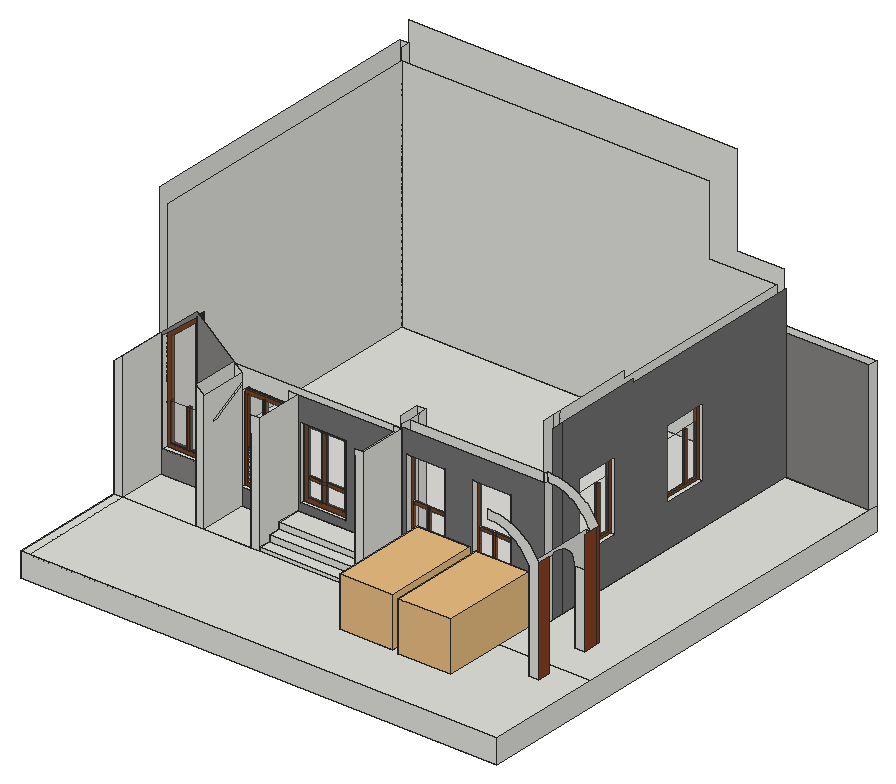
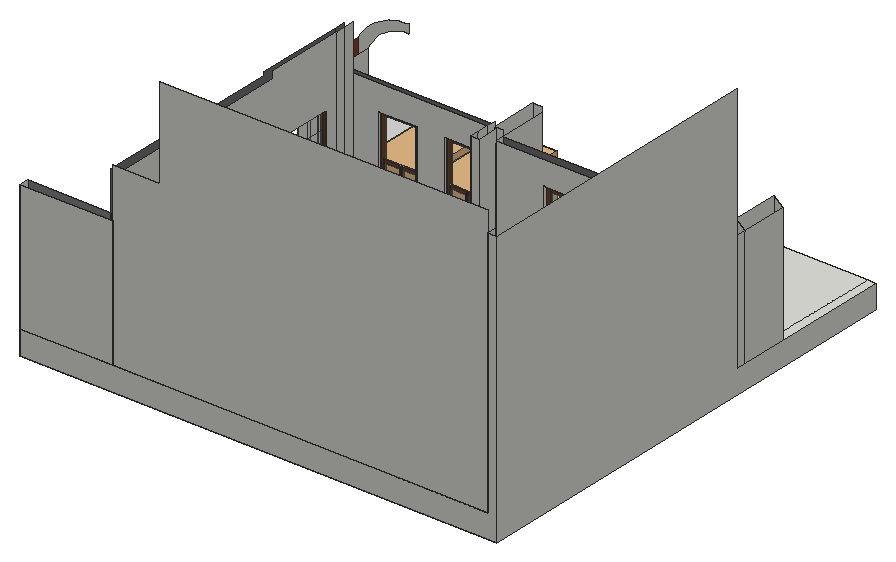
# SketchUp Ruby script. Lengths in inches.
U = 1.inch
M = Sketchup.active_model
def pt(a) = Geom::Point3d.new(a.map { |v| v * U })
def face(e, loops, mat)
  f = e.add_face(loops[0].map { |a| pt(a) })
  loops[1..].each { |l| e.add_face(l.map { |a| pt(a) }).erase! }
  f.material = f.back_material = mat if mat
  f
end
# faces: each face lists its corners as indices into pts; further lists are holes
def faces(e, pts, list, mat = nil) = list.each { |f| face(e, (f[0].is_a?(Array) ? f : [f]).map { |l| l.map { |i| pts[i] } }, mat) }
# xy, xz, yz: faces in a plane at the given z, y or x. An outline is a flat list of corners, or four numbers for a rectangle; further outlines are holes
def ring(l) = l.size == 4 ? [[l[0], l[1]], [l[2], l[1]], [l[2], l[3]], [l[0], l[3]]] : l.each_slice(2).to_a
def flat(e, list, mat, &to3) = list.each { |f| face(e, (f[0].is_a?(Array) ? f : [f]).map { |l| ring(l).map { |u, v| to3.(u, v) } }, mat) }
def xy(e, z, list, mat = nil) = flat(e, list, mat) { |x, y| [x, y, z] }
def xz(e, y, list, mat = nil) = flat(e, list, mat) { |x, z| [x, y, z] }
def yz(e, x, list, mat = nil) = flat(e, list, mat) { |y, z| [x, y, z] }
def lines(e, pts, list) = list.each { |a, b| e.add_line(pt(pts[a]), pt(pts[b])) }
# prism: a flat outline (further loops are holes) pulled along v
def prism(e, loops, v, mat = nil)
  f = face(e, loops, mat); d = Geom::Vector3d.new(v.map { |x| x * U })
  f.pushpull(f.normal.samedirection?(d) ? d.length : -d.length)
end
def box(e, o, s, mat = nil) = prism(e, [[o, [o[0] + s[0], o[1], o[2]], [o[0] + s[0], o[1] + s[1], o[2]], [o[0], o[1] + s[1], o[2]]]], [0, 0, s[2]], mat)
def at(x, y, z, deg = 0) = Geom::Transformation.translation(pt([x, y, z])) * Geom::Transformation.rotation(ORIGIN, Z_AXIS, deg.degrees)
def axes(o, x, y, z) = Geom::Transformation.new([*x, 0, *y, 0, *z, 0, *pt(o).to_a, 1])
def part(name) = M.definitions.add(name)
# library, detail: a bought-in or finely detailed component or shape, given as its bounding box
def library(name, o, s) = part(name).tap { |d| box(d.entities, o, s) }
def detail(e, o, s) = box(e.add_group.entities, o, s)
def put(e, d, t, mat = nil) = e.add_instance(d, t).tap { |i| i.material = mat if mat }
def group(e, t, mat = nil) = e.add_group.tap { |g| g.transformation = t; g.material = mat if mat }.entities
root = M.entities
M.materials.add("Glass Thin Clear 001").color = [243, 240, 240]
M.materials["Glass Thin Clear 001"].alpha = 0.1
M.materials.add("[Brick Tumbled]").color = [135, 132, 132]
M.materials.add("[Color M05]").color = [114, 114, 114]
M.materials.add("[Roofing Tile Spanish]").color = [138, 64, 36]
M.materials.add("[Wood Veneer 01]").color = [120, 70, 37]
c1 = library("2016+Honda+Civic+LX+Sedan",[0.01,0.03,0.02],[16.17,34.46,10.62])
xy(root,-24,[[9.96,0,489.96,478.0625]])
xy(root,0,[[9.96,0,18.96,118.0625],[[18.96,0,489.96,118.0625],[446.88,93.6875,457.27,105.875]],[446.88,93.6875,457.27,105.875],[9.96,118.0625,18.96,166.0625],[18.96,118.0625,91.87,166.0625],
  [91.87,118.0625,156.96,166.0625],[91.87,118.0625,99.96,166.0625],[99.96,118.0625,147.96,166.0625],[147.96,118.0625,156.96,166.0625],[156.96,118.0625,252.96,166.0625],
  [252.96,118.0625,261.96,166.0625],[[261.96,118.0625,489.96,118.0625,489.96,469.0625,405.96,469.0625,405.96,166.0625,261.96,166.0625],[446.88,151.74,457.27,169.5]],[446.88,151.74,457.27,166.0625],[9.96,166.0625,18.96,175.0625],[18.96,166.0625,252.96,175.0625],
  [252.96,166.0625,261.96,196.0625],[252.96,166.0625,405.96,166.0625,405.96,469.0625,396.96,469.0625,396.96,196.0625,252.96,196.0625],[261.96,166.0625,405.96,175.0625],[446.88,166.0625,457.27,169.5],[446.88,166.0625,457.27,169.5],
  [18.96,175.0625,252.96,175.0625,252.96,196.0625,396.96,196.0625,396.96,469.0625,18.96,469.0625],[261.96,175.0625,396.96,187.0625],[396.96,175.0625,405.96,187.0625],[261.96,187.0625,396.96,196.0625],[396.96,187.0625,405.96,469.0625],
  [18.96,469.0625,396.96,478.0625],[396.96,469.0625,489.96,478.0625]])
xy(root,3.4375,[[156.96,118.0625,252.96,129.9375]])
xy(root,9.4375,[[156.96,129.9375,252.96,142.0625]])
xy(root,15.4375,[[156.96,142.0625,252.96,166.0625]])
xy(root,16.69,[[99.96,166.0625,147.96,170.5625],[99.96,173.4375,147.96,175.0625]])
xy(root,16.69,[[99.96,170.5625,147.96,172.375],[99.96,172.375,147.96,173.4375]],"[Wood Veneer 01]")
xy(root,19.54,[[102.81,170.5625,117.68,171.125],[117.68,170.5625,120.35,173.4375],[120.35,170.5625,145.12,171.125]])
xy(root,19.54,[[102.81,171.125,117.68,173.4375],[120.35,171.125,145.12,173.4375]],"[Wood Veneer 01]")
xy(root,22.88,[[159.41,166.0625,204.66,170.5625],[159.41,170.5625,204.66,171.8125],[159.41,171.8125,204.66,172.375],[159.41,172.375,204.66,175.0625]])
xy(root,23.7,[[21.04,166.0625,54.79,170.5625],[21.04,173.875,54.79,175.0625]])
xy(root,23.7,[[21.04,170.5625,54.79,171.0625],[21.04,171.0625,54.79,173.0625],[21.04,173.0625,54.79,173.875]],"[Wood Veneer 01]")
xy(root,27.23,[[177.76,170.5625,182.03,172.375]])
xy(root,27.23,[[163.76,170.5625,177.76,170.875],[182.03,170.5625,200.3125,170.875],[163.76,170.875,177.76,172.375],[182.03,170.875,200.3125,172.375]],"[Wood Veneer 01]")
xy(root,27.76,[[41.61,170.5625,44.06,171.0625],[41.61,171.0625,44.06,173.875]])
xy(root,27.76,[[25.1,170.5625,41.61,171.0625],[44.06,170.5625,50.73,171.0625],[25.1,171.0625,41.61,173.875],[44.06,171.0625,50.73,173.875]],"[Wood Veneer 01]")
xy(root,31.4,[[266.93,166.0625,304.99,170.5625],[333.18,166.0625,371.24,170.5625],[266.93,172.1875,304.99,175.0625],[333.18,172.1875,371.24,175.0625]])
xy(root,31.4,[[266.93,170.5625,304.99,171.8125],[333.18,170.5625,371.24,171.8125],[266.93,171.8125,304.99,172.1875],[333.18,171.8125,371.24,172.1875]],"[Wood Veneer 01]")
xy(root,34.51,[[283.58,170.5625,285.96,172.1875],[349.83,170.5625,352.21,172.1875]])
xy(root,34.51,[[270.03,170.5625,283.58,170.875],[285.96,170.5625,301.89,170.875],[336.28,170.5625,349.83,170.875],[352.21,170.5625,368.14,170.875],[270.03,170.875,283.58,172.1875],
  [285.96,170.875,301.89,172.1875],[336.28,170.875,349.83,172.1875],[352.21,170.875,368.14,172.1875]],"[Wood Veneer 01]")
xy(root,42.82,[[396.96,208.32,398.84,253.94],[398.84,208.32,400.59,253.94],[400.59,208.32,401.46,253.94],[401.46,208.32,405.96,253.94],[396.96,318.94,398.84,364.57],
  [398.84,318.94,400.59,364.57],[400.59,318.94,401.46,364.57],[401.46,318.94,405.96,364.57]])
xy(root,44.17,[[163.76,170.5625,177.76,170.875],[177.76,170.5625,182.03,172.375],[182.03,170.5625,200.3125,170.875],[163.76,170.875,177.76,172.375],[182.03,170.875,200.3125,172.375]])
xy(root,44.65,[[398.84,237.2,401.46,239.92],[398.84,347.83,401.46,350.54]])
xy(root,44.65,[[398.84,210.14,399.27,237.2],[399.27,210.14,401.46,237.2],[398.84,239.92,399.27,252.12],[399.27,239.92,401.46,252.12],[398.84,320.77,399.27,347.83],
  [399.27,320.77,401.46,347.83],[398.84,350.54,399.27,362.74],[399.27,350.54,401.46,362.74]],"[Wood Veneer 01]")
xy(root,47.11,[[177.76,170.5625,182.03,172.375]])
xy(root,47.11,[[163.76,170.5625,177.76,170.875],[182.03,170.5625,200.3125,170.875],[163.76,170.875,177.76,172.375],[182.03,170.875,200.3125,172.375]],"[Wood Veneer 01]")
xy(root,49.23,[[117.68,170.5625,120.35,173.4375]])
xy(root,49.23,[[102.81,170.5625,117.68,171.125],[120.35,170.5625,145.12,171.125],[102.81,171.125,117.68,173.4375],[120.35,171.125,145.12,173.4375]],"[Wood Veneer 01]")
xy(root,52.125,[[117.68,170.5625,120.35,173.4375]])
xy(root,52.125,[[102.81,170.5625,117.68,171.125],[120.35,170.5625,145.12,171.125],[102.81,171.125,117.68,173.4375],[120.35,171.125,145.12,173.4375]],"[Wood Veneer 01]")
xy(root,58.94,[[283.58,170.5625,285.96,172.1875],[349.83,170.5625,352.21,172.1875]])
xy(root,58.94,[[270.03,170.5625,283.58,170.875],[285.96,170.5625,301.89,170.875],[336.28,170.5625,349.83,170.875],[352.21,170.5625,368.14,170.875],[270.03,170.875,283.58,172.1875],
  [285.96,170.875,301.89,172.1875],[336.28,170.875,349.83,172.1875],[352.21,170.875,368.14,172.1875]],"[Wood Veneer 01]")
xz(root,0,[[9.96,-24,489.96,0]])
xz(root,93.6875,[[446.88,0,457.27,0,457.27,105.64,454.61,110.13,451.55,114.36,448.11,118.29,444.67,121.5625,444.33,121.88,440.24,125.125,435.87,127.97,431.26,130.42,430.75,130.625,426.4375,132.43,421.46,133.99,416.36,135.09,411.18,135.72,405.96,135.875,405.96,127.6,410.3125,127.28,414.61,126.55,418.82,125.42,422.91,123.88,426.82,121.97,427.48,121.5625,430.54,119.68,434.02,117.06,437.24,114.11,440.16,110.87,442.75,107.36,445,103.62,446.88,99.6875]])
xz(root,105.875,[[446.88,0,457.27,73.29]])
xz(root,118.0625,[[9.96,0,18.96,0,18.96,127.72,9.96,120],[91.87,0,99.96,0,99.96,120,91.87,127.08],[147.96,0,156.96,120],[156.96,0,252.96,3.4375],[252.96,0,261.96,126]])
xz(root,129.9375,[[156.96,3.4375,252.96,9.4375]])
xz(root,142.0625,[[156.96,9.4375,252.96,15.4375]])
xz(root,151.74,[[446.88,0,457.27,73.29]])
xz(root,166.0625,[[9.96,0,9.96,120,18.96,127.72,18.96,0],[91.87,0,91.87,127.08,99.96,120,99.96,0],[147.96,0,156.96,120],[156.96,0,252.96,15.4375],[252.96,0,261.96,126],
  [446.88,0,457.27,99.6875]])
xz(root,166.0625,[[[18.96,0,91.87,0,91.87,127.08,55.42,159,18.96,127.72],[21.04,23.7,21.04,126.39,54.79,154.64,54.79,23.7]]],"[Brick Tumbled]")
xz(root,166.0625,[[99.96,0,147.96,16.69],[[261.96,0,405.96,127.6],[266.93,31.4,304.99,105.09],[333.18,31.4,371.24,105.09]],[[156.96,15.4375,252.96,120],[159.41,22.88,204.66,96.1]]],"[Color M05]")
xz(root,169.5,[[446.88,0,446.88,99.6875,445,103.62,442.75,107.36,440.16,110.87,437.24,114.11,434.02,117.06,430.54,119.68,427.48,121.5625,426.82,121.97,422.91,123.88,418.82,125.42,414.61,126.55,410.3125,127.28,405.96,127.6,405.96,135.875,411.18,135.72,416.36,135.09,421.46,133.99,426.4375,132.43,430.75,130.625,431.26,130.42,435.87,127.97,440.24,125.125,444.33,121.88,444.67,121.5625,448.11,118.29,451.55,114.36,454.61,110.13,457.27,105.64,457.27,0]])
xz(root,170.5625,[[[99.96,16.69,147.96,102.98],[102.81,19.54,145.12,100.14]],[117.68,19.54,120.35,49.23],[[159.41,22.88,204.66,96.1],[163.76,27.23,200.3125,91.75]],[[21.04,23.7,54.79,23.7,54.79,154.64,21.04,126.39],[25.1,27.76,25.1,124.49,41.61,138.3,44.06,140.36,50.73,145.9375,50.73,27.76]],[177.76,27.23,182.03,44.17],
  [41.61,27.76,44.06,66.22],[[266.93,31.4,304.99,105.09],[270.03,34.51,301.89,101.99]],[[333.18,31.4,371.24,105.09],[336.28,34.51,368.14,101.99]],[283.58,34.51,285.96,58.94],[349.83,34.51,352.21,58.94],
  [163.76,44.17,177.76,47.11],[177.76,44.17,182.03,47.11],[182.03,44.17,200.3125,47.11],[177.76,47.11,182.03,91.75],[102.81,49.23,117.68,52.125],
  [117.68,49.23,120.35,52.125],[120.35,49.23,145.12,52.125],[117.68,52.125,120.35,100.14],[270.03,58.94,283.58,61.76],[283.58,58.94,285.96,61.76],
  [285.96,58.94,301.89,61.76],[336.28,58.94,349.83,61.76],[349.83,58.94,352.21,61.76],[352.21,58.94,368.14,61.76]],"[Wood Veneer 01]")
xz(root,170.875,[[163.76,27.23,177.76,44.17],[182.03,27.23,200.3125,44.17],[270.03,34.51,283.58,58.94],[285.96,34.51,301.89,58.94],[336.28,34.51,349.83,58.94],
  [352.21,34.51,368.14,58.94],[163.76,47.11,177.76,91.75],[182.03,47.11,200.3125,91.75]],"Glass Thin Clear 001")
xz(root,171.0625,[[[21.04,23.7,21.04,126.39,54.79,154.64,54.79,23.7],[25.1,27.76,50.73,27.76,50.73,145.9375,44.06,140.36,41.61,138.3,25.1,124.49]],[41.61,27.76,44.06,66.22]])
xz(root,171.0625,[[25.1,27.76,41.61,66.22],[44.06,27.76,50.73,66.22]],"Glass Thin Clear 001")
xz(root,171.125,[[102.81,19.54,117.68,49.23],[120.35,19.54,145.12,49.23],[102.81,52.125,117.68,100.14],[120.35,52.125,145.12,100.14]],"Glass Thin Clear 001")
xz(root,171.8125,[[159.41,22.88,204.66,96.1],[266.93,31.4,304.99,105.09],[333.18,31.4,371.24,105.09]],"Glass Thin Clear 001")
xz(root,172.1875,[[[266.93,31.4,304.99,105.09],[270.03,34.51,301.89,101.99]],[[333.18,31.4,371.24,105.09],[336.28,34.51,368.14,101.99]],[283.58,34.51,285.96,58.94],[349.83,34.51,352.21,58.94],[270.03,58.94,283.58,61.76],
  [283.58,58.94,285.96,61.76],[285.96,58.94,301.89,61.76],[336.28,58.94,349.83,61.76],[349.83,58.94,352.21,61.76],[352.21,58.94,368.14,61.76]],"[Wood Veneer 01]")
xz(root,172.375,[[99.96,16.69,147.96,102.98]],"Glass Thin Clear 001")
xz(root,172.375,[[[159.41,22.88,204.66,96.1],[163.76,27.23,200.3125,91.75]],[177.76,27.23,182.03,44.17],[163.76,44.17,177.76,47.11],[177.76,44.17,182.03,47.11],[182.03,44.17,200.3125,47.11],
  [177.76,47.11,182.03,91.75]],"[Wood Veneer 01]")
xz(root,173.0625,[[21.04,23.7,21.04,126.39,54.79,154.64,54.79,23.7]],"Glass Thin Clear 001")
xz(root,173.4375,[[[99.96,16.69,147.96,102.98],[102.81,19.54,145.12,100.14]],[117.68,19.54,120.35,49.23],[102.81,49.23,117.68,52.125],[117.68,49.23,120.35,52.125],[120.35,49.23,145.12,52.125],
  [117.68,52.125,120.35,100.14]],"[Wood Veneer 01]")
xz(root,173.875,[[[21.04,23.7,21.04,126.39,54.79,154.64,54.79,23.7],[25.1,27.76,50.73,27.76,50.73,145.9375,44.06,140.36,41.61,138.3,25.1,124.49]],[41.61,27.76,44.06,66.22]],"[Wood Veneer 01]")
xz(root,175.0625,[[9.96,0,18.96,120],[[18.96,0,18.96,120,21.04,120,21.04,23.7,54.79,23.7,54.79,120,252.96,120,252.96,0],[99.96,16.69,147.96,102.98],[159.41,22.88,204.66,96.1]],[[261.96,0,396.96,130.625],[333.18,31.4,371.24,105.09],[266.93,31.4,304.99,105.09]],[396.96,0,405.96,130.625]])
xz(root,196.0625,[[252.96,0,261.96,130.625]])
xz(root,208.32,[[396.96,42.82,398.84,112.57],[401.46,42.82,405.96,112.57]])
xz(root,208.32,[[398.84,42.82,400.59,112.57],[400.59,42.82,401.46,112.57]],"[Wood Veneer 01]")
xz(root,210.14,[[398.84,44.65,399.27,93.98],[399.27,44.65,401.46,93.98]],"[Wood Veneer 01]")
xz(root,237.2,[[398.84,44.65,399.27,93.98],[399.27,44.65,401.46,93.98]],"[Wood Veneer 01]")
xz(root,239.92,[[398.84,44.65,399.27,93.98],[399.27,44.65,401.46,93.98]],"[Wood Veneer 01]")
xz(root,252.12,[[398.84,44.65,399.27,93.98],[399.27,44.65,401.46,93.98]],"[Wood Veneer 01]")
xz(root,253.94,[[396.96,42.82,398.84,112.57],[401.46,42.82,405.96,112.57]])
xz(root,253.94,[[398.84,42.82,400.59,112.57],[400.59,42.82,401.46,112.57]],"[Wood Veneer 01]")
xz(root,318.94,[[396.96,42.82,398.84,112.57],[401.46,42.82,405.96,112.57]])
xz(root,318.94,[[398.84,42.82,400.59,112.57],[400.59,42.82,401.46,112.57]],"[Wood Veneer 01]")
xz(root,320.77,[[398.84,44.65,399.27,93.98],[399.27,44.65,401.46,93.98]],"[Wood Veneer 01]")
xz(root,347.83,[[398.84,44.65,399.27,93.98],[399.27,44.65,401.46,93.98]],"[Wood Veneer 01]")
xz(root,350.54,[[398.84,44.65,399.27,93.98],[399.27,44.65,401.46,93.98]],"[Wood Veneer 01]")
xz(root,362.74,[[398.84,44.65,399.27,93.98],[399.27,44.65,401.46,93.98]],"[Wood Veneer 01]")
xz(root,364.57,[[396.96,42.82,398.84,112.57],[401.46,42.82,405.96,112.57]])
xz(root,364.57,[[398.84,42.82,400.59,112.57],[400.59,42.82,401.46,112.57]],"[Wood Veneer 01]")
xz(root,469.0625,[[18.96,0,396.96,0,396.96,170.02,328.85,170.02,328.85,240,18.96,240],[396.96,0,405.96,130.625]])
xz(root,469.0625,[[405.96,0,489.96,130.625]],"[Brick Tumbled]")
xz(root,478.0625,[[9.96,-24,9.96,252,18.96,252,18.96,0,489.96,0,489.96,-24],[18.96,0,18.96,272.68,348.92,272.68,348.92,180.58,396.96,180.58,396.96,0],[396.96,0,489.96,130.625]])
yz(root,9.96,[[0,-24,0,0,175.0625,0,175.0625,252,478.0625,252,478.0625,-24],[118.0625,0,166.0625,120],[166.0625,0,175.0625,120]])
yz(root,18.96,[[118.0625,0,166.0625,127.72],[175.0625,0,469.0625,240],[469.0625,0,478.0625,252]])
yz(root,21.04,[[166.0625,23.7,170.5625,126.39],[173.875,23.7,175.0625,126.39]])
yz(root,21.04,[[170.5625,23.7,171.0625,126.39],[171.0625,23.7,173.0625,126.39],[173.0625,23.7,173.875,126.39]],"[Wood Veneer 01]")
yz(root,25.1,[[170.5625,27.76,171.0625,66.22],[171.0625,27.76,173.875,66.22]],"[Wood Veneer 01]")
yz(root,41.61,[[170.5625,27.76,171.0625,66.22],[171.0625,27.76,173.875,66.22]],"[Wood Veneer 01]")
yz(root,44.06,[[170.5625,27.76,171.0625,66.22],[171.0625,27.76,173.875,66.22]],"[Wood Veneer 01]")
yz(root,50.73,[[170.5625,27.76,171.0625,66.22],[171.0625,27.76,173.875,66.22]],"[Wood Veneer 01]")
yz(root,54.79,[[166.0625,23.7,170.5625,154.64],[173.875,23.7,175.0625,154.64]])
yz(root,54.79,[[170.5625,23.7,171.0625,154.64],[171.0625,23.7,173.0625,154.64],[173.0625,23.7,173.875,154.64]],"[Wood Veneer 01]")
yz(root,91.87,[[118.0625,0,166.0625,127.08]])
yz(root,99.96,[[118.0625,0,166.0625,0,166.0625,107.76,143.8,95.875,135.72,91.5625,127.4375,91.5625,135.72,95.875,166.0625,111.67,166.0625,120,118.0625,120],[166.0625,16.69,170.5625,102.98],[173.4375,16.69,175.0625,102.98]])
yz(root,99.96,[[170.5625,16.69,172.375,102.98],[172.375,16.69,173.4375,102.98]],"[Wood Veneer 01]")
yz(root,102.81,[[171.125,19.54,173.4375,49.23],[170.5625,49.23,173.4375,52.125]])
yz(root,102.81,[[170.5625,19.54,171.125,49.23],[170.5625,52.125,171.125,100.14],[171.125,52.125,173.4375,100.14]],"[Wood Veneer 01]")
yz(root,117.68,[[170.5625,49.23,173.4375,52.125]])
yz(root,117.68,[[170.5625,19.54,171.125,49.23],[171.125,19.54,173.4375,49.23],[170.5625,52.125,171.125,100.14],[171.125,52.125,173.4375,100.14]],"[Wood Veneer 01]")
yz(root,120.35,[[170.5625,19.54,171.125,49.23],[171.125,19.54,173.4375,49.23],[170.5625,49.23,173.4375,52.125]])
yz(root,120.35,[[170.5625,52.125,171.125,100.14],[171.125,52.125,173.4375,100.14]],"[Wood Veneer 01]")
yz(root,145.12,[[170.5625,49.23,173.4375,52.125]])
yz(root,145.12,[[170.5625,19.54,171.125,49.23],[171.125,19.54,173.4375,49.23],[170.5625,52.125,171.125,100.14],[171.125,52.125,173.4375,100.14]],"[Wood Veneer 01]")
yz(root,147.96,[[118.0625,0,166.0625,16.69],[118.0625,16.69,118.0625,102.98,149.375,102.98,135.72,95.875,127.4375,91.5625,135.72,91.5625,143.8,95.875,157.11,102.98,166.0625,102.98,166.0625,16.69],[166.0625,16.69,170.5625,102.98],[173.4375,16.69,175.0625,102.98]])
yz(root,147.96,[[170.5625,16.69,172.375,102.98],[172.375,16.69,173.4375,102.98]],"[Wood Veneer 01]")
yz(root,156.96,[[118.0625,0,118.0625,3.4375,129.9375,3.4375,129.9375,9.4375,142.0625,9.4375,142.0625,15.4375,166.0625,15.4375,166.0625,0],[118.0625,3.4375,129.9375,3.4375,129.9375,9.4375,142.0625,9.4375,142.0625,15.4375,166.0625,15.4375,166.0625,120,118.0625,120]])
yz(root,159.41,[[166.0625,22.88,170.5625,96.1],[172.375,22.88,175.0625,96.1]])
yz(root,159.41,[[170.5625,22.88,171.8125,96.1],[171.8125,22.88,172.375,96.1]],"[Wood Veneer 01]")
yz(root,163.76,[[170.5625,44.17,172.375,47.11]])
yz(root,163.76,[[170.5625,27.23,170.875,44.17],[170.875,27.23,172.375,44.17],[170.5625,47.11,170.875,91.75],[170.875,47.11,172.375,91.75]],"[Wood Veneer 01]")
yz(root,177.76,[[170.5625,44.17,172.375,47.11]])
yz(root,177.76,[[170.5625,27.23,170.875,44.17],[170.875,27.23,172.375,44.17],[170.5625,47.11,170.875,91.75],[170.875,47.11,172.375,91.75]],"[Wood Veneer 01]")
yz(root,182.03,[[170.5625,44.17,172.375,47.11]])
yz(root,182.03,[[170.5625,27.23,170.875,44.17],[170.875,27.23,172.375,44.17],[170.5625,47.11,170.875,91.75],[170.875,47.11,172.375,91.75]],"[Wood Veneer 01]")
yz(root,200.3125,[[170.5625,44.17,172.375,47.11]])
yz(root,200.3125,[[170.5625,27.23,170.875,44.17],[170.875,27.23,172.375,44.17],[170.5625,47.11,170.875,91.75],[170.875,47.11,172.375,91.75]],"[Wood Veneer 01]")
yz(root,204.66,[[166.0625,22.88,170.5625,96.1],[172.375,22.88,175.0625,96.1]])
yz(root,204.66,[[170.5625,22.88,171.8125,96.1],[171.8125,22.88,172.375,96.1]],"[Wood Veneer 01]")
yz(root,252.96,[[166.0625,0,175.0625,120],[175.0625,0,196.0625,130.625],[118.0625,3.4375,118.0625,120,166.0625,120,166.0625,15.4375,142.0625,15.4375,142.0625,9.4375,129.9375,9.4375,129.9375,3.4375]])
yz(root,261.96,[[118.0625,0,166.0625,126],[166.0625,0,175.0625,130.625],[175.0625,0,187.0625,130.625],[187.0625,0,196.0625,130.625]])
yz(root,266.93,[[166.0625,31.4,170.5625,105.09],[172.1875,31.4,175.0625,105.09]])
yz(root,266.93,[[170.5625,31.4,171.8125,105.09],[171.8125,31.4,172.1875,105.09]],"[Wood Veneer 01]")
yz(root,270.03,[[170.5625,58.94,172.1875,61.76]])
yz(root,270.03,[[170.5625,34.51,170.875,58.94],[170.875,34.51,172.1875,58.94]],"[Wood Veneer 01]")
yz(root,283.58,[[170.5625,58.94,172.1875,61.76]])
yz(root,283.58,[[170.5625,34.51,170.875,58.94],[170.875,34.51,172.1875,58.94]],"[Wood Veneer 01]")
yz(root,285.96,[[170.5625,58.94,172.1875,61.76]])
yz(root,285.96,[[170.5625,34.51,170.875,58.94],[170.875,34.51,172.1875,58.94]],"[Wood Veneer 01]")
yz(root,301.89,[[170.5625,58.94,172.1875,61.76]])
yz(root,301.89,[[170.5625,34.51,170.875,58.94],[170.875,34.51,172.1875,58.94]],"[Wood Veneer 01]")
yz(root,304.99,[[166.0625,31.4,170.5625,105.09],[172.1875,31.4,175.0625,105.09]])
yz(root,304.99,[[170.5625,31.4,171.8125,105.09],[171.8125,31.4,172.1875,105.09]],"[Wood Veneer 01]")
yz(root,333.18,[[166.0625,31.4,170.5625,105.09],[172.1875,31.4,175.0625,105.09]])
yz(root,333.18,[[170.5625,31.4,171.8125,105.09],[171.8125,31.4,172.1875,105.09]],"[Wood Veneer 01]")
yz(root,336.28,[[170.5625,58.94,172.1875,61.76]])
yz(root,336.28,[[170.5625,34.51,170.875,58.94],[170.875,34.51,172.1875,58.94]],"[Wood Veneer 01]")
yz(root,349.83,[[170.5625,58.94,172.1875,61.76]])
yz(root,349.83,[[170.5625,34.51,170.875,58.94],[170.875,34.51,172.1875,58.94]],"[Wood Veneer 01]")
yz(root,352.21,[[170.5625,58.94,172.1875,61.76]])
yz(root,352.21,[[170.5625,34.51,170.875,58.94],[170.875,34.51,172.1875,58.94]],"[Wood Veneer 01]")
yz(root,368.14,[[170.5625,58.94,172.1875,61.76]])
yz(root,368.14,[[170.5625,34.51,170.875,58.94],[170.875,34.51,172.1875,58.94]],"[Wood Veneer 01]")
yz(root,371.24,[[166.0625,31.4,170.5625,105.09],[172.1875,31.4,175.0625,105.09]])
yz(root,371.24,[[170.5625,31.4,171.8125,105.09],[171.8125,31.4,172.1875,105.09]],"[Wood Veneer 01]")
yz(root,396.96,[[175.0625,0,187.0625,177],[187.0625,0,196.0625,177],[[196.0625,0,196.0625,177,276.6875,177,276.6875,170.02,469.0625,170.02,469.0625,0],[208.32,42.82,253.94,112.57],[318.94,42.82,364.57,112.57]],[469.0625,0,478.0625,130.625]])
yz(root,398.84,[[[208.32,42.82,253.94,112.57],[210.14,44.65,252.12,110.75]],[[318.94,42.82,364.57,112.57],[320.77,44.65,362.74,110.75]],[237.2,44.65,239.92,93.98],[347.83,44.65,350.54,93.98]],"[Wood Veneer 01]")
yz(root,399.27,[[210.14,44.65,237.2,93.98],[239.92,44.65,252.12,93.98],[320.77,44.65,347.83,93.98],[350.54,44.65,362.74,93.98]],"Glass Thin Clear 001")
yz(root,400.59,[[208.32,42.82,253.94,112.57],[318.94,42.82,364.57,112.57]],"Glass Thin Clear 001")
yz(root,401.46,[[[208.32,42.82,253.94,112.57],[210.14,44.65,252.12,110.75]],[[318.94,42.82,364.57,112.57],[320.77,44.65,362.74,110.75]],[237.2,44.65,239.92,93.98],[347.83,44.65,350.54,93.98]],"[Wood Veneer 01]")
yz(root,405.96,[[166.0625,0,175.0625,0,175.0625,130.625,169.5,130.625,169.5,127.6,166.0625,127.6]])
yz(root,405.96,[[175.0625,0,187.0625,173],[[187.0625,0,469.0625,0,469.0625,170.02,276.6875,170.02,276.6875,173,187.0625,173],[318.94,42.82,364.57,112.57],[208.32,42.82,253.94,112.57]]],"[Color M05]")
yz(root,446.88,[[93.6875,0,93.6875,99.6875,166.0625,99.6875,166.0625,0,151.74,0,151.74,75.78,151.64,77.02,151.47,78.25,151.24,79.47,150.93,80.68,150.57,81.86,150.14,83.03,149.65,84.17,149.09,85.29,148.48,86.37,147.8125,87.41,147.09,88.42,146.31,89.39,145.48,90.32,144.6,91.2,143.67,92.02,142.7,92.8,141.69,93.53,140.64,94.2,139.5625,94.81,138.45,95.36,137.31,95.85,136.14,96.28,134.95,96.64,133.74,96.94,132.52,97.18,131.29,97.35,130.05,97.45,128.81,97.48,127.57,97.45,126.33,97.35,125.1,97.18,123.875,96.94,122.67,96.64,121.48,96.28,120.3125,95.85,119.17,95.36,118.06,94.81,116.98,94.2,115.93,93.53,114.92,92.8,113.95,92.02,113.02,91.2,112.14,90.32,111.3125,89.39,110.53,88.42,109.81,87.41,109.14,86.37,108.53,85.29,107.97,84.17,107.48,83.03,107.05,81.86,106.68,80.68,106.38,79.47,106.15,78.25,105.98,77.02,105.88,75.78,105.875,75.69,105.875,0],[166.0625,0,169.5,99.6875]])
yz(root,457.27,[[93.6875,0,105.875,0,105.875,73.29,105.84,74.54,105.875,75.69,105.875,105.64,93.6875,105.64],[151.74,0,166.0625,0,166.0625,105.64,151.74,105.64,151.74,75.69,151.78,74.54,151.74,73.29],[166.0625,0,169.5,105.64]],"[Roofing Tile Spanish]")
yz(root,489.96,[[0,-24,478.0625,0],[469.0625,0,478.0625,130.625]])
put(root,c1,axes([397.64,155.79,-0.1],[-3.29,0,0],[0,-2.84612,0],[0,0,4.65]))
put(root,c1,axes([283.79,59.62,-0.08],[3.29,0,0],[0,2.84612,0],[0,0,4.65]))
